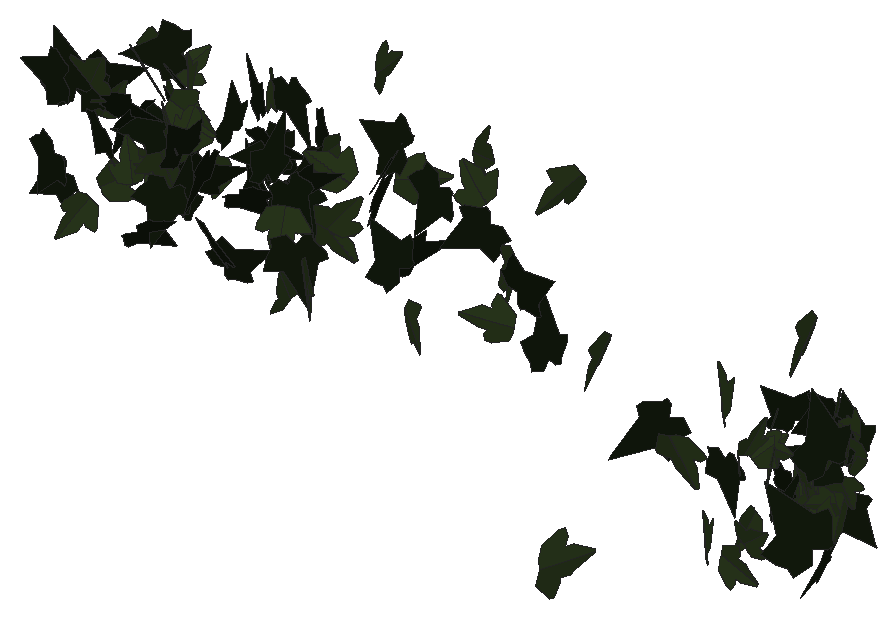
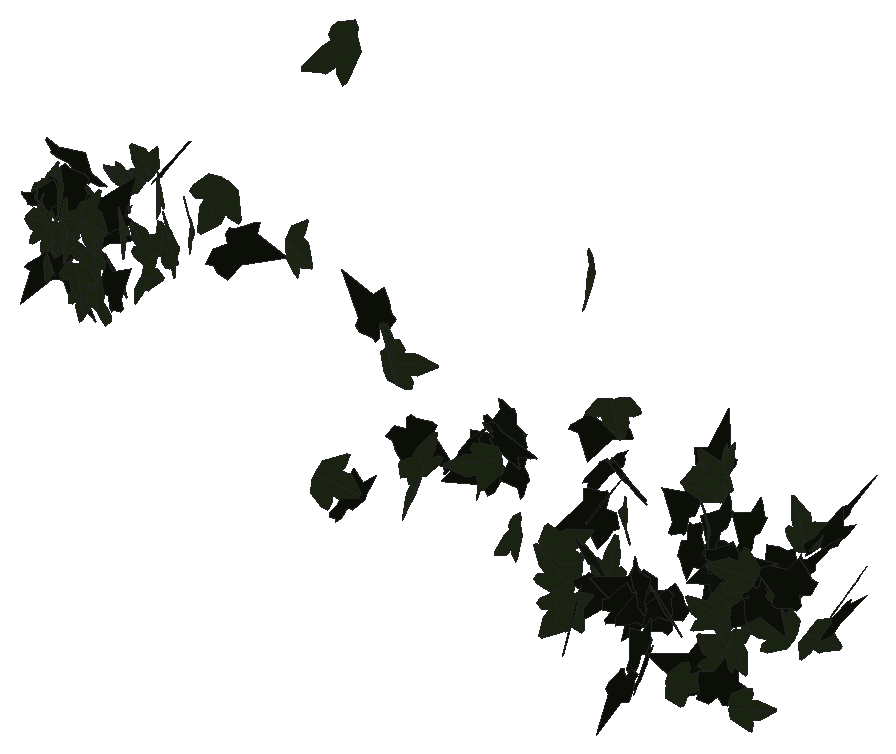
# SketchUp Ruby script. Lengths in inches.
U = 1.inch
M = Sketchup.active_model
def pt(a) = Geom::Point3d.new(a.map { |v| v * U })
def face(e, loops, mat)
  f = e.add_face(loops[0].map { |a| pt(a) })
  loops[1..].each { |l| e.add_face(l.map { |a| pt(a) }).erase! }
  f.material = f.back_material = mat if mat
  f
end
# faces: each face lists its corners as indices into pts; further lists are holes
def faces(e, pts, list, mat = nil) = list.each { |f| face(e, (f[0].is_a?(Array) ? f : [f]).map { |l| l.map { |i| pts[i] } }, mat) }
# xy, xz, yz: faces in a plane at the given z, y or x. An outline is a flat list of corners, or four numbers for a rectangle; further outlines are holes
def ring(l) = l.size == 4 ? [[l[0], l[1]], [l[2], l[1]], [l[2], l[3]], [l[0], l[3]]] : l.each_slice(2).to_a
def flat(e, list, mat, &to3) = list.each { |f| face(e, (f[0].is_a?(Array) ? f : [f]).map { |l| ring(l).map { |u, v| to3.(u, v) } }, mat) }
def xy(e, z, list, mat = nil) = flat(e, list, mat) { |x, y| [x, y, z] }
def xz(e, y, list, mat = nil) = flat(e, list, mat) { |x, z| [x, y, z] }
def yz(e, x, list, mat = nil) = flat(e, list, mat) { |y, z| [x, y, z] }
def lines(e, pts, list) = list.each { |a, b| e.add_line(pt(pts[a]), pt(pts[b])) }
# prism: a flat outline (further loops are holes) pulled along v
def prism(e, loops, v, mat = nil)
  f = face(e, loops, mat); d = Geom::Vector3d.new(v.map { |x| x * U })
  f.pushpull(f.normal.samedirection?(d) ? d.length : -d.length)
end
def box(e, o, s, mat = nil) = prism(e, [[o, [o[0] + s[0], o[1], o[2]], [o[0] + s[0], o[1] + s[1], o[2]], [o[0], o[1] + s[1], o[2]]]], [0, 0, s[2]], mat)
def at(x, y, z, deg = 0) = Geom::Transformation.translation(pt([x, y, z])) * Geom::Transformation.rotation(ORIGIN, Z_AXIS, deg.degrees)
def axes(o, x, y, z) = Geom::Transformation.new([*x, 0, *y, 0, *z, 0, *pt(o).to_a, 1])
def part(name) = M.definitions.add(name)
# library, detail: a bought-in or finely detailed component or shape, given as its bounding box
def library(name, o, s) = part(name).tap { |d| box(d.entities, o, s) }
def detail(e, o, s) = box(e.add_group.entities, o, s)
def put(e, d, t, mat = nil) = e.add_instance(d, t).tap { |i| i.material = mat if mat }
def group(e, t, mat = nil) = e.add_group.tap { |g| g.transformation = t; g.material = mat if mat }.entities
root = M.entities
M.materials.add("efeu1").color = [18, 25, 13]
M.materials.add("efeu2").color = [43, 57, 29]
c1 = part("ivyleaf_9")
p = [[1.54,2.16,1.25],[1.36,2.04,1.19],[-0.21,0.99,0.68],[-0.71,1.11,0.82],[-0.85,0.86,0.67],[-0.8,0.17,0.21],
  [-0.9,-0.01,0.1],[-0.67,-0.16,-0.02],[-0.08,-0.08,-0.05],[-0.03,-0.6,-0.4],[0.65,-0.88,-0.66],[0.83,-0.6,-0.49],
  [1.29,-0.42,-0.43],[1.8125,-0.07,-0.26],[1.21,0.44,0.15]]
faces(c1.entities,p,[[0,1,2,3,4,5,6,7,8,9,10,11,12,13,14]],"efeu1")
c2 = part("ivyleaf_10")
p = [[0,0.5,-0.03],[-0.0625,2.02,-0.43],[-0.19,2.01,-0.46],[-0.54,1.05,-0.29],[-0.52,0.625,-0.18],[-0.83,0.76,-0.28],
  [-1.16,0.64,-0.33],[-1.15,0.33,-0.24],[-0.77,-0.39,0.02],[-0.3,-0.51,0.16],[0.04,-0.48,0.23],[-0.02,2.01,-0.4375],
  [-0.06,2.01,-0.43],[0.04,-0.49,0.23],[0.67,-0.49,0.14],[1.38,0.36,-0.2],[1.375,0.51,-0.24],[0.81,0.65,-0.19],
  [0.62,0.59,-0.15],[0.6,1.09,-0.28],[0.5,1.23,-0.31]]
faces(c2.entities,p,[[0,1,2,3,4,5,6,7,8,9,10],[11,12,0,13,14,15,16,17,18,19,20]],"efeu2")
put(root,c1,axes([541.87,131.67,162.86],[-0.47307,-0.69223,0.34621],[0.19735,0.28447,0.83843],[-0.7484,0.51258,0.00225]))
put(root,c2,axes([542.23,136.71,157.18],[-0.06014,-0.01271,-0.78677],[-0.78371,-0.06974,0.06103],[-0.07051,0.78598,-0.0073]))
put(root,c1,axes([541.81,130.83,163.59],[0.15613,-0.8369,-0.20601],[0.09793,-0.19078,0.84925],[-0.8563,-0.17441,0.05956]))
put(root,c1,axes([541.95,133.23,162.13],[-0.03417,-0.74609,-0.23376],[0.03791,-0.23528,0.74543],[-0.78093,0.02123,0.04641]))
put(root,c1,axes([541.55,130.62,159.93],[-0.0403,-0.66265,0.60596],[0.02044,-0.60709,-0.66252],[0.8977,-0.01593,0.04229]))
put(root,c1,axes([541.22,134.14,161.87],[0.09938,-0.0196,0.83537],[0.80722,-0.21511,-0.10108],[0.2159,0.81329,-0.00661]))
put(root,c1,axes([541.77,131.06,158.9],[0.26408,-0.46942,-0.61497],[0.28801,-0.54346,0.5385],[-0.71805,-0.39062,-0.01017]))
put(root,c2,axes([542.25,133.33,161.11],[-0.26804,-0.65007,0.30384],[0.12527,0.27697,0.7031],[-0.70655,0.29572,0.0094]))
put(root,c2,axes([542.4,132.14,163.12],[-0.80953,-0.05323,0.43726],[0.43862,-0.01318,0.81044],[-0.04055,0.91998,0.03691]))
put(root,c2,axes([542.95,130.9,157.84],[0.30455,0.47978,-0.64791],[-0.34167,-0.55052,-0.56826],[-0.73023,0.45768,-0.00433]))
put(root,c2,axes([542.57,135.9,162.98],[-0.17566,-0.28464,0.76462],[0.47142,0.60295,0.33276],[-0.6659,0.50194,0.03388]))
put(root,c2,axes([542.99,136.15,159.63],[0.14602,-0.75395,0.32438],[0.09247,-0.31227,-0.76741],[0.81554,0.1704,0.02893]))
put(root,c1,axes([542.59,132.47,160.73],[0.52201,-0.30648,-0.677],[0.58834,-0.33499,0.6053],[-0.45399,-0.78652,0.006]))
put(root,c1,axes([543.35,133.93,161.14],[-0.23147,0.56882,-0.55447],[0.21795,-0.50989,-0.61407],[-0.76386,-0.31785,-0.00719]))
put(root,c1,axes([542.72,132.93,161.8],[0.66555,0.04328,0.44833],[0.44625,0.04515,-0.66682],[-0.0611,0.80119,0.01336]))
put(root,c1,axes([543.9,136.04,163.2],[-0.49449,-0.09724,0.67365],[-0.65303,-0.16694,-0.50345],[0.19187,-0.81881,0.02264]))
put(root,c1,axes([543.45,136.57,157.36],[0.34089,0.25534,0.67418],[-0.54715,-0.39395,0.42586],[0.46941,-0.64462,0.00679]))
put(root,c2,axes([543.05,137.24,161.5],[0.4347,0.27046,-0.61403],[0.51203,0.33909,0.51185],[0.43359,-0.67158,0.01115]))
put(root,c2,axes([542.96,136.77,160.21],[-0.25788,0.06992,0.74698],[0.72601,-0.17588,0.2671],[0.18915,0.77042,-0.00682]))
put(root,c2,axes([543.375,132.27,158.44],[-0.11865,-0.32298,0.86052],[0.31509,0.80079,0.34401],[-0.86344,0.33661,0.00729]))
put(root,c1,axes([544.02,134.8,160.17],[-0.0308,-0.60233,-0.52802],[-0.02642,-0.52736,0.60312],[-0.80057,0.04058,0.00041]))
put(root,c2,axes([543.95,132.77,158.9375],[0.22503,0.77662,-0.08698],[-0.00167,0.09099,0.80812],[0.78147,-0.22344,0.02677]))
put(root,c2,axes([543.76,135.86,158.65],[-0.17007,-0.65855,0.49115],[0.09944,0.48137,0.67987],[-0.81549,0.19604,-0.01953]))
put(root,c1,axes([543.89,133.74,163.55],[0.30961,-0.49402,0.63243],[0.35243,-0.5253,-0.58287],[0.72098,0.46892,0.01333]))
put(root,c1,axes([544.25,135.26,162.64],[0.68245,-0.45545,0.16105],[0.13595,-0.08641,-0.82047],[0.46356,0.69586,0.00352]))
put(root,c2,axes([545.2,137.25,157.47],[0.0282,0.00844,-0.81112],[-0.58651,-0.56045,-0.02622],[-0.56035,0.58703,-0.01338]))
put(root,c2,axes([545.35,133.19,160],[-0.57437,-0.67103,-0.23331],[0.14252,0.18508,-0.88321],[0.69599,-0.59167,-0.01168]))
put(root,c1,axes([544.72,136.0625,157.51],[0.24522,-0.05088,0.81395],[0.8155,0.02395,-0.24419],[-0.0083,0.84975,0.05562]))
put(root,c2,axes([546.14,134,163.24],[0.33739,-0.2002,0.78548],[-0.65245,0.43781,0.39184],[-0.48102,-0.73427,0.01947]))
put(root,c1,axes([546.49,136.42,160.39],[-0.65025,0.31147,-0.4384],[-0.4178,0.14052,0.71954],[0.3386,0.77154,0.04593]))
put(root,c1,axes([546.41,139.1875,158.13],[0.196,-0.26161,-0.79321],[-0.48122,0.63057,-0.32688],[0.68268,0.5196,-0.00268]))
put(root,c1,axes([546.16,133.12,162.625],[0.37002,-0.60724,0.58866],[0.27697,-0.5201,-0.71061],[0.7991,0.46144,-0.02628]))
put(root,c1,axes([547.1875,137.28,161.21],[0.07164,-0.16404,0.80507],[-0.28384,0.75343,0.17878],[-0.77103,-0.2926,0.00899]))
put(root,c1,axes([546.67,129.99,158.33],[0.55055,0.60789,0.21632],[0.13887,0.16607,-0.8201],[-0.63012,0.56773,0.00827]))
put(root,c1,axes([546.9375,132.36,158.4375],[-0.31879,-0.39713,0.63358],[0.42211,0.47294,0.50883],[-0.61722,0.52856,0.02075]))
put(root,c1,axes([546.89,131.56,159.64],[-0.47736,-0.66946,-0.11372],[0.06901,0.09046,-0.82221],[0.67553,-0.48231,0.00364]))
put(root,c1,axes([547.13,137.2,157.08],[0.01992,-0.60547,0.55825],[0.06895,0.55768,0.60239],[-0.82066,0.03216,0.06416]))
put(root,c1,axes([547.2,137.08,158.18],[0.1992,-0.46664,0.64707],[0.27073,-0.58781,-0.50725],[0.75043,0.33593,0.01124]))
put(root,c2,axes([548.5625,129.91,163.18],[-0.60231,0.5595,-0.36444],[-0.26934,0.24553,0.82208],[0.611,0.65978,0.00312]))
put(root,c1,axes([548.27,132.52,161.15],[-0.32842,0.29888,-0.74763],[0.52419,-0.53351,-0.44355],[-0.61115,-0.61821,0.02133]))
put(root,c2,axes([547.6,131.375,163.95],[0.3413,0.13266,0.88613],[0.82395,0.3261,-0.36617],[-0.35205,0.89184,0.00208]))
put(root,c1,axes([548.7,136.97,159.68],[-0.26521,-0.21482,0.76067],[-0.60341,-0.46324,-0.3412],[0.51056,-0.65907,-0.00812]))
put(root,c2,axes([548.13,131.16,162.83],[0.80467,0.10699,-0.20891],[0.20615,0.03455,0.81172],[0.11222,-0.83063,0.00685]))
put(root,c1,axes([547.89,136.31,160.25],[0.48435,0.23023,-0.68763],[0.61566,0.30638,0.53623],[0.38316,-0.78331,0.00763]))
put(root,c1,axes([548.93,133.92,159.1],[0.6286,0.53932,0.06963],[0.04349,0.05624,-0.82813],[-0.54205,0.62994,0.01432]))
put(root,c1,axes([549.08,129.79,163.01],[0.28177,0.37491,0.77182],[-0.43537,-0.63757,0.46864],[0.7394,-0.51828,-0.01819]))
put(root,c2,axes([548.69,136.15,163.31],[0.09407,-0.03316,0.82359],[0.72168,-0.39717,-0.09842],[0.39823,0.72761,-0.01619]))
put(root,c1,axes([549.49,138.37,160.62],[0.3803,-0.18969,-0.73007],[-0.64684,0.3386,-0.42492],[0.38804,0.75032,0.00718]))
put(root,c2,axes([550.28,138.34,159.86],[-0.05212,0.12562,-0.83945],[-0.27183,-0.79921,-0.10272],[-0.80409,0.26204,0.08914]))
put(root,c1,axes([549.64,132.07,156.85],[0.03646,-0.05868,0.82497],[0.79736,-0.21681,-0.05066],[0.21965,0.79681,0.04697]))
put(root,c1,axes([550.18,135.55,163.93],[0.39228,-0.79365,-0.08846],[-0.03247,0.08262,-0.88527],[0.7979,0.39355,0.00747]))
put(root,c1,axes([550.76,135.22,159.39],[-0.35526,-0.45486,-0.67218],[0.42287,0.52255,-0.5771],[0.69275,-0.55224,0.00757]))
put(root,c1,axes([551.65,135.16,160.73],[-0.69488,0.55146,0.08852],[-0.07371,0.04951,-0.88709],[-0.55364,-0.69874,0.007]))
put(root,c2,axes([551.72,139.66,163.59],[0.01001,-0.12864,-0.89619],[0.04206,0.89534,-0.12804],[0.9044,-0.04022,0.01587]))
put(root,c1,axes([551.1,129.12,159.875],[0.2869,-0.41934,0.71364],[0.43867,-0.56347,-0.50746],[0.70193,0.52354,0.02545]))
put(root,c1,axes([552.01,131.86,162.27],[-0.73865,0.49497,0.09156],[0.07102,-0.05847,0.88911],[0.49833,0.74201,0.00899]))
put(root,c2,axes([552.82,135.64,160.65],[0.39042,0.36257,0.70909],[-0.5411,-0.45868,0.53246],[0.58436,-0.66697,0.01928]))
put(root,c2,axes([552.375,135.56,157.98],[-0.73728,-0.21023,-0.44186],[0.42959,0.10451,-0.76652],[0.2343,-0.85317,0.01499]))
put(root,c1,axes([552.61,132.77,161.24],[-0.02666,0.44524,-0.77119],[-0.17375,0.75411,0.44138],[0.87338,0.16361,0.06427]))
put(root,c2,axes([553.04,134.95,158.77],[-0.5516,-0.49762,0.50713],[0.38483,0.33044,0.74282],[-0.59725,0.6725,0.01026]))
put(root,c2,axes([553.52,131.42,157.11],[-0.13985,-0.72219,-0.46884],[-0.08779,-0.46055,0.73561],[-0.85654,0.16512,0.00115]))
put(root,c1,axes([553.65,131.21,162.36],[0.23419,-0.67682,-0.46544],[-0.13482,0.44576,-0.71603],[0.81028,0.26979,0.01539]))
put(root,c2,axes([555.76,128.125,163.04],[0.75487,0.49216,-0.09203],[-0.07741,-0.04977,-0.90114],[-0.49467,0.75883,0.00059]))
put(root,c1,axes([556.93,134.53,163.93],[-0.5721,-0.13817,-0.71312],[-0.69401,-0.16401,0.58855],[-0.21444,0.89941,-0.00223]))
put(root,c1,axes([556.875,132.79,161.82],[0.02685,0.27281,0.86951],[0.15748,0.85541,-0.27325],[-0.89759,0.15824,-0.02193]))
put(root,c1,axes([556.55,128.05,161.92],[-0.33337,-0.6476,-0.54356],[0.2502,0.48255,-0.72836],[0.80761,-0.41681,0.00128]))
put(root,c1,axes([557.37,132.74,163.59],[-0.42199,0.62784,-0.45369],[-0.30158,0.34272,0.75478],[0.71349,0.5162,0.0507]))
put(root,c2,axes([557.28,134.47,162.66],[-0.04066,-0.07681,-0.92279],[0.776,0.50114,-0.0759],[0.50523,-0.77591,0.04232]))
put(root,c2,axes([558.55,137.71,162.8],[-0.22696,0.46707,0.73714],[-0.37113,0.63769,-0.51832],[-0.7898,-0.43387,0.03174]))
put(root,c1,axes([558.74,134.71,162.55],[-0.15285,-0.77773,0.5064],[-0.07278,-0.5016,-0.79232],[0.92521,-0.16794,0.02133]))
put(root,c1,axes([560.07,130.4,161.18],[-0.81342,-0.06509,-0.4059],[-0.40207,-0.06147,0.8156],[-0.08563,0.90698,0.02615]))
put(root,c1,axes([559.33,131.59,160.6875],[0.34661,0.42746,0.77907],[0.47725,0.61586,-0.55024],[-0.74961,0.58975,0.00992]))
put(root,c2,axes([559.92,136.05,162.08],[0.20682,0.83198,0.2688],[-0.07932,-0.25722,0.85718],[0.87072,-0.22105,0.01424]))
put(root,c2,axes([561.07,129.92,159.37],[-0.41109,0.78469,0.13375],[-0.06514,0.11687,-0.88585],[-0.79334,-0.4162,0.00343]))
put(root,c1,axes([561.97,133.99,162.27],[0.06247,0.05227,-0.90793],[-0.60107,-0.68058,-0.08054],[-0.68248,0.60419,-0.01218]))
put(root,c2,axes([561.45,122.55,164.82],[-0.34025,0.59912,-0.75382],[0.36547,-0.65932,-0.68898],[-0.89085,-0.49931,0.00526]))
put(root,c2,axes([562.24,139.24,162.17],[-0.09481,-0.54965,0.7909],[-0.14676,-0.77719,-0.55773],[0.95189,-0.17458,-0.00721]))
put(root,c1,axes([565.375,133.73,157.35],[-0.33794,-0.61115,0.6123],[0.29807,0.53485,0.69836],[-0.81214,0.45061,0.00153]))
put(root,c2,axes([566.33,130.06,163.52],[0.55045,-0.60703,-0.60546],[-0.38388,0.46885,-0.81907],[0.76662,0.67064,0.02459]))
put(root,c2,axes([566.84,128.92,161.47],[0.13119,0.09856,0.91362],[-0.75689,-0.51174,0.16389],[0.52108,-0.76814,0.00805]))
put(root,c1,axes([567.57,129.0625,163.24],[-0.00766,0.02402,0.95368],[0.69763,-0.65036,0.02198],[0.65069,0.69756,-0.01235]))
put(root,c2,axes([573.81,126.87,163.8],[0.29176,-0.70339,0.62013],[0.22697,-0.57717,-0.76145],[0.90984,0.36954,-0.00891]))
put(root,c1,axes([577.82,126.07,162.05],[-0.00627,-0.12235,-0.99511],[0.04712,-0.99406,0.12193],[-1.00149,-0.046,0.01197]))
put(root,c2,axes([579.36,128.04,162.26],[0.50073,-0.28781,0.93325],[-0.81894,0.44766,0.57745],[-0.53209,-0.95984,-0.01052]))
put(root,c2,axes([580.21,123.71,162.7],[-1.01179,0.03262,-0.302],[0.30186,-0.00923,-1.01232],[-0.0339,-1.05586,-0.00049]))
put(root,c2,axes([580.65,131.99,164.76],[0.27151,-0.58831,0.83544],[0.38229,-0.74316,-0.64757],[0.94759,0.46838,0.02188]))
put(root,c2,axes([581.82,128.29,162.86],[0.2594,-0.56888,-0.52076],[-0.21702,0.47339,-0.62523],[0.74008,0.33821,-0.00081]))
put(root,c1,axes([582.25,128.49,159.21],[0.19118,-0.29055,0.70837],[-0.37564,0.6006,0.34773],[-0.66715,-0.42143,0.0072]))
put(root,c1,axes([582.55,128.59,162.67],[0.28256,0.11286,0.72381],[-0.69499,-0.20393,0.30311],[0.23157,-0.74977,0.02651]))
put(root,c2,axes([582.42,126.01,158.875],[0.05738,0.45285,-0.71624],[-0.07868,-0.71193,-0.45643],[-0.84373,0.09719,-0.00614]))
put(root,c2,axes([583.03,122.26,159.45],[0.32556,-0.21101,0.84982],[-0.72394,0.44517,0.38787],[-0.49258,-0.79373,-0.00838]))
put(root,c2,axes([583.07,128.59,160.76],[-0.65011,0.15279,0.20239],[-0.1964,0.04893,-0.66782],[-0.16041,-0.67913,-0.00258]))
put(root,c2,axes([583.19,124.1,162.1],[0.16453,-0.35192,-0.67997],[-0.25502,0.63059,-0.38807],[0.72192,0.30296,0.01789]))
put(root,c2,axes([583.14,128.42,158.46],[1.09419,-0.24456,0.466],[-0.44855,0.12893,1.12089],[-0.27526,-1.18227,0.02584]))
put(root,c1,axes([583.09,126.95,159.02],[-0.38113,0.63616,0.26285],[0.12355,-0.23235,0.74148],[0.67714,0.40046,0.01266]))
put(root,c2,axes([583.26,124.77,163.15],[-0.04767,-0.67232,0.28148],[0.03295,0.27981,0.6739],[-0.72812,0.05668,0.01207]))
put(root,c1,axes([583.03,123.42,163.06],[0.22174,-0.81171,0.07205],[0.02134,-0.06886,-0.84145],[0.81462,0.22275,0.00243]))
put(root,c2,axes([583.19,111.53,163.4],[-0.04846,-0.19143,-1.2224],[0.46986,1.12885,-0.19541],[1.14461,-0.47149,0.02846]))
put(root,c2,axes([583.45,129.09,160.16],[0.69904,0.11114,-0.07676],[-0.10257,0.17357,-0.68283],[-0.08788,0.68149,0.18643]))
put(root,c2,axes([583.66,127.63,160.91],[-0.5863,0.39386,-0.08414],[0.06995,-0.04676,-0.70631],[-0.39663,-0.59046,-0.00019]))
put(root,c2,axes([583.41,125.26,162.72],[0.29778,0.19412,-0.5897],[0.45474,0.37705,0.35376],[0.42266,-0.54244,0.03486]))
put(root,c2,axes([583.6,125.87,162.47],[0.39199,-0.43666,0.27965],[0.19713,-0.19876,-0.58666],[0.4796,0.43859,0.01256]))
put(root,c2,axes([583.74,128.72,162.42],[0.06213,0.28714,-0.62811],[0.09526,0.62106,0.29333],[0.68403,-0.11257,0.0162]))
put(root,c2,axes([583.5,124.36,158.93],[-0.51592,-0.09188,0.56594],[0.56748,0.02683,0.52168],[-0.08183,0.76534,0.04965]))
put(root,c2,axes([584.02,128.05,158.62],[-0.24979,-0.59166,-0.09975],[0.04026,0.09127,-0.64223],[0.59866,-0.25301,0.00157]))
put(root,c2,axes([583.9,127.91,159.58],[0.00227,0.00279,0.67476],[0.22409,-0.63647,0.00188],[0.63646,0.22409,-0.00307]))
put(root,c2,axes([583.58,125.78,162.96],[0.01791,-0.04334,-0.66126],[0.61206,-0.25248,0.03312],[-0.25401,-0.61143,0.0332]))
put(root,c2,axes([583.44,123.08,158.55],[0.17873,-0.001,0.83864],[0.83116,0.11451,-0.177],[-0.11178,0.84979,0.02484]))
put(root,c1,axes([584.85,128.41,163.6],[0.04932,0.15495,-0.96836],[-0.8308,-0.50855,-0.12369],[-0.52105,0.82554,0.10556]))
put(root,c2,axes([584.39,128.54,162.4],[0.14307,-0.86044,-0.56095],[-0.0801,0.55529,-0.87219],[1.02401,0.16365,0.01015]))
put(root,c2,axes([584.9,128.45,163.31],[-0.02312,0.07791,0.97058],[-0.70803,0.66513,-0.07026],[-0.66843,-0.70722,0.04085]))
put(root,c2,axes([585.41,127.46,160.11],[-0.21519,-0.05753,0.63415],[-0.60435,-0.19237,-0.22253],[0.20055,-0.64144,0.00986]))
put(root,c1,axes([585.56,127.75,161.84],[-0.29741,0.01344,0.79495],[-0.79473,-0.02946,-0.29683],[0.02289,-0.84825,0.0229]))
put(root,c2,axes([585.32,127.27,162.625],[-0.29563,-0.63879,-0.07901],[0.0329,0.07183,-0.70388],[0.64282,-0.29745,-0.00031]))
put(root,c1,axes([585.63,128.6875,162.4],[-0.75733,-0.18452,0.12875],[0.12703,0.0225,0.77944],[-0.18571,0.76787,0.0081]))
put(root,c1,axes([586.17,125.14,159.33],[-0.95684,-0.57871,-0.15269],[-0.12537,-0.08774,1.11819],[-0.58524,0.96497,0.01011]))
put(root,c1,axes([586.2,126.26,163.11],[-1.05106,0.09283,-0.25707],[-0.25606,0.02271,1.05515],[0.09556,1.0818,-0.0001]))
put(root,c2,axes([585.67,128.77,161.54],[0.22189,-0.44936,0.6347],[-0.26155,0.57846,0.50098],[-0.73237,-0.34273,0.01338]))
put(root,c1,axes([585.9,126.66,158.04],[-0.59559,0.46518,-0.28155],[0.22215,-0.17298,-0.75572],[-0.4963,-0.63567,-0.00039]))
put(root,c2,axes([585.51,128.04,159.85],[-0.06731,-0.82149,0.45825],[0.2919,-0.45499,-0.77276],[0.89422,0.08669,0.28674]))
put(root,c2,axes([585.625,128.04,160.89],[-0.61421,-0.23064,-0.13414],[0.12556,0.04719,-0.65609],[0.23542,-0.62691,-0.00004]))
put(root,c2,axes([585.88,128.23,162.82],[-0.66147,-0.00829,0.20409],[-0.20378,-0.02059,-0.6613],[0.01399,-0.69193,0.01724]))
put(root,c2,axes([585.67,128.75,162.98],[-0.15065,0.48791,0.4801],[0.13942,-0.45942,0.51064],[0.67016,0.20526,0.00169]))
put(root,c1,axes([585.47,128.29,159.61],[0.07249,-0.45219,-0.68465],[-0.06266,0.68226,-0.45725],[0.8181,0.09232,0.02564]))
put(root,c2,axes([585.6,128.71,162.5625],[-0.23236,0.29228,0.69124],[0.34496,-0.60105,0.3701],[0.66652,0.41297,0.04943]))
